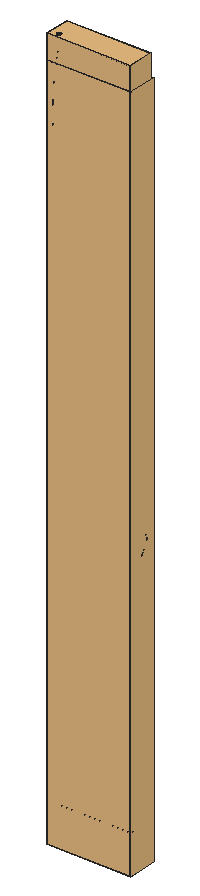
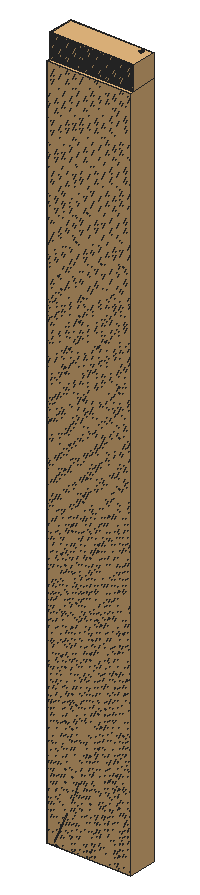
# SketchUp Ruby script. Lengths in inches.
U = 1.inch
M = Sketchup.active_model
def pt(a) = Geom::Point3d.new(a.map { |v| v * U })
def face(e, loops, mat)
  f = e.add_face(loops[0].map { |a| pt(a) })
  loops[1..].each { |l| e.add_face(l.map { |a| pt(a) }).erase! }
  f.material = f.back_material = mat if mat
  f
end
# faces: each face lists its corners as indices into pts; further lists are holes
def faces(e, pts, list, mat = nil) = list.each { |f| face(e, (f[0].is_a?(Array) ? f : [f]).map { |l| l.map { |i| pts[i] } }, mat) }
# xy, xz, yz: faces in a plane at the given z, y or x. An outline is a flat list of corners, or four numbers for a rectangle; further outlines are holes
def ring(l) = l.size == 4 ? [[l[0], l[1]], [l[2], l[1]], [l[2], l[3]], [l[0], l[3]]] : l.each_slice(2).to_a
def flat(e, list, mat, &to3) = list.each { |f| face(e, (f[0].is_a?(Array) ? f : [f]).map { |l| ring(l).map { |u, v| to3.(u, v) } }, mat) }
def xy(e, z, list, mat = nil) = flat(e, list, mat) { |x, y| [x, y, z] }
def xz(e, y, list, mat = nil) = flat(e, list, mat) { |x, z| [x, y, z] }
def yz(e, x, list, mat = nil) = flat(e, list, mat) { |y, z| [x, y, z] }
def lines(e, pts, list) = list.each { |a, b| e.add_line(pt(pts[a]), pt(pts[b])) }
# prism: a flat outline (further loops are holes) pulled along v
def prism(e, loops, v, mat = nil)
  f = face(e, loops, mat); d = Geom::Vector3d.new(v.map { |x| x * U })
  f.pushpull(f.normal.samedirection?(d) ? d.length : -d.length)
end
def box(e, o, s, mat = nil) = prism(e, [[o, [o[0] + s[0], o[1], o[2]], [o[0] + s[0], o[1] + s[1], o[2]], [o[0], o[1] + s[1], o[2]]]], [0, 0, s[2]], mat)
def at(x, y, z, deg = 0) = Geom::Transformation.translation(pt([x, y, z])) * Geom::Transformation.rotation(ORIGIN, Z_AXIS, deg.degrees)
def axes(o, x, y, z) = Geom::Transformation.new([*x, 0, *y, 0, *z, 0, *pt(o).to_a, 1])
def part(name) = M.definitions.add(name)
# library, detail: a bought-in or finely detailed component or shape, given as its bounding box
def library(name, o, s) = part(name).tap { |d| box(d.entities, o, s) }
def detail(e, o, s) = box(e.add_group.entities, o, s)
def put(e, d, t, mat = nil) = e.add_instance(d, t).tap { |i| i.material = mat if mat }
def group(e, t, mat = nil) = e.add_group.tap { |g| g.transformation = t; g.material = mat if mat }.entities
root = M.entities
M.materials.add("green").color = [174, 139, 102]
c1 = library("3DGeom~169_Defintion",[-36.08,-38.12,-500],[72.16,76.24,1000])
c2 = part("3DGeom~170_Defintion")
p = [[22.63,21.29,-499.8],[10.94,15.58,-499.92],[15.89,19.76,-500],[22.63,21.29,-499.8],[9.12,9.86,-499.6],[10.94,15.58,-499.92],
  [22.63,21.29,-499.8],[22.56,-1.57,-498.16],[15.83,-0.04,-498.58],[22.63,21.29,-499.8],[29.3,-0.04,-497.96],[22.56,-1.57,-498.16],
  [22.63,21.29,-499.8],[15.83,-0.04,-498.58],[10.91,4.15,-499.1],[22.63,21.29,-499.8],[34.25,4.15,-498.04],[29.3,-0.04,-497.96],
  [22.63,21.29,-499.8],[10.91,4.15,-499.1],[9.12,9.86,-499.6],[22.63,21.29,-499.8],[36.08,9.86,-498.37],[34.25,4.15,-498.04],
  [22.63,21.29,-499.8],[34.29,15.58,-498.86],[36.08,9.86,-498.37],[22.63,21.29,-499.8],[29.37,19.76,-499.39],[34.29,15.58,-498.86],
  [-22.3,-38.12,487.14],[-22.89,-17.99,500],[-34.125,-33.09,489.82],[-22.3,-38.12,487.14],[-34.125,-33.09,489.82],[-29.08,-36.77,487.69],
  [-10.78,-33.09,490.89],[-22.89,-17.99,500],[-22.3,-38.12,487.14],[-10.78,-33.09,490.89],[-22.3,-38.12,487.14],[-15.6,-36.77,488.31],
  [-34.125,-33.09,489.82],[-34.42,-23.02,496.25],[-36.08,-28.06,492.96],[-34.125,-33.09,489.82],[-22.89,-17.99,500],[-34.42,-23.02,496.25],
  [-11.07,-23.02,497.32],[-22.89,-17.99,500],[-10.78,-33.09,490.89],[-11.07,-23.02,497.32],[-10.78,-33.09,490.89],[-9.12,-28.06,494.18],
  [-22.89,-17.99,500],[-29.59,-19.34,498.83],[-34.42,-23.02,496.25],[-22.89,-17.99,500],[-11.07,-23.02,497.32],[-16.11,-19.34,499.45]]
faces(c2.entities,p,[[0,1,2],[3,4,5],[6,7,8],[9,10,11],[12,13,14],[15,16,17],[18,19,20],[21,22,23],
  [24,25,26],[27,28,29],[30,31,32],[33,34,35],[36,37,38],[39,40,41],[42,43,44],[45,46,47],
  [48,49,50],[51,52,53],[54,55,56],[57,58,59]],"green")
c3 = library("3DGeom~69_Defintion",[-21.55,-528.54,-60.47],[37.16,1000,121.53])
c4 = library("3DGeom~67_Defintion",[-21.08,-482.92,-59.16],[42.16,1000,118.9])
c5 = library("3DGeom~72_Defintion",[-21.55,-528.54,-60.94],[37.16,1000,122])
c6 = library("3DGeom~71_Defintion",[-21.08,-482.92,-59.62],[42.16,1000,119.36])
c7 = part("3DGeom~73_Defintion")
p = [[11.99,496.51,-49.8],[15.53,496.29,-49.63],[13.73,496.34,-49.94],[11.99,496.51,-49.8],[19.55,496.875,-46.43],[15.53,496.29,-49.63],
  [8.98,497.16,-48.31],[19.55,496.875,-46.43],[11.99,496.51,-49.8],[8.98,497.16,-48.31],[11.99,496.51,-49.8],[10.38,496.79,-49.24],
  [15.53,496.29,-49.63],[19.55,496.875,-46.43],[18.54,496.57,-47.79],[15.53,496.29,-49.63],[18.54,496.57,-47.79],[17.18,496.37,-48.89],
  [7.13,498.09,-45.48],[19.55,496.875,-46.43],[8.98,497.16,-48.31],[7.13,498.09,-45.48],[8.98,497.16,-48.31],[7.87,497.6,-47.04],
  [7.06,499.03,-42.12],[19.55,496.875,-46.43],[7.13,498.09,-45.48],[8.7,499.72,-39.2],[19.55,496.875,-46.43],[7.06,499.03,-42.12],
  [11.72,500,-37.36],[19.55,496.875,-46.43],[8.7,499.72,-39.2],[15.25,499.78,-37.19],[19.55,496.875,-46.43],[11.72,500,-37.36],
  [20.18,497.26,-44.875],[19.55,496.875,-46.43],[15.25,499.78,-37.19],[7.06,499.03,-42.12],[7.13,498.09,-45.48],[6.86,498.58,-43.78],
  [20.18,497.26,-44.875],[15.25,499.78,-37.19],[16.86,499.5,-37.75],[19.37,498.7,-39.95],[20.18,497.26,-44.875],[16.86,499.5,-37.75],
  [20.11,498.2,-41.51],[20.18,497.26,-44.875],[19.37,498.7,-39.95],[20.11,498.2,-41.51],[20.38,497.71,-43.21],[20.18,497.26,-44.875],
  [8.7,499.72,-39.2],[7.06,499.03,-42.12],[7.6875,499.41,-40.5625],[19.37,498.7,-39.95],[16.86,499.5,-37.75],[18.26,499.13,-38.68],
  [11.72,500,-37.36],[8.7,499.72,-39.2],[10.0625,499.92,-38.11],[15.25,499.78,-37.19],[11.72,500,-37.36],[13.51,499.95,-37.05],
  [-14.64,-499.34,43.17],[-13.98,-499.3,43.1],[-13.3,-499.28,43.21],[-15.79,-499.47,43.77],[-15.26,-499.4,43.4],[-14.64,-499.34,43.17],
  [-15.79,-499.47,43.77],[-14.64,-499.34,43.17],[-11.78,-499.375,44.44],[-14.64,-499.34,43.17],[-13.3,-499.28,43.21],[-11.78,-499.375,44.44],
  [-13.3,-499.28,43.21],[-12.16,-499.32,43.91],[-11.78,-499.375,44.44],[-13.3,-499.28,43.21],[-12.68,-499.29,43.49],[-12.16,-499.32,43.91],
  [-16.49,-499.66,44.89],[-16.21,-499.56,44.28],[-15.79,-499.47,43.77],[-16.49,-499.66,44.89],[-15.79,-499.47,43.77],[-11.78,-499.375,44.44],
  [-15.9,-499.96,47.36],[-16.52,-499.84,46.22],[-11.78,-499.375,44.44],[-14.76,-500,48.06],[-15.9,-499.96,47.36],[-11.78,-499.375,44.44],
  [-13.42,-499.94,48.1],[-14.76,-500,48.06],[-11.78,-499.375,44.44],[-11.54,-499.44,45.05],[-13.42,-499.94,48.1],[-11.78,-499.375,44.44],
  [-16.52,-499.84,46.22],[-16.49,-499.66,44.89],[-11.78,-499.375,44.44],[-16.52,-499.84,46.22],[-16.6,-499.75,45.57],[-16.49,-499.66,44.89],
  [-11.54,-499.44,45.05],[-12.81,-499.88,47.87],[-13.42,-499.94,48.1],[-11.85,-499.72,46.99],[-12.81,-499.88,47.87],[-11.54,-499.44,45.05],
  [-11.54,-499.44,45.05],[-11.57,-499.625,46.375],[-11.85,-499.72,46.99],[-11.54,-499.44,45.05],[-11.47,-499.53,45.7],[-11.57,-499.625,46.375],
  [-15.9,-499.96,47.36],[-16.28,-499.91,46.83],[-16.52,-499.84,46.22],[-11.85,-499.72,46.99],[-12.28,-499.81,47.5],[-12.81,-499.88,47.87],
  [-14.76,-500,48.06],[-15.39,-499.99,47.78],[-15.9,-499.96,47.36],[-13.42,-499.94,48.1],[-14.08,-499.98,48.17],[-14.76,-500,48.06]]
faces(c7.entities,p,[[0,1,2],[3,4,5],[6,7,8],[9,10,11],[12,13,14],[15,16,17],[18,19,20],[21,22,23],
  [24,25,26],[27,28,29],[30,31,32],[33,34,35],[36,37,38],[39,40,41],[42,43,44],[45,46,47],
  [48,49,50],[51,52,53],[54,55,56],[57,58,59],[60,61,62],[63,64,65],[66,67,68],[69,70,71],
  [72,73,74],[75,76,77],[78,79,80],[81,82,83],[84,85,86],[87,88,89],[90,91,92],[93,94,95],
  [96,97,98],[99,100,101],[102,103,104],[105,106,107],[108,109,110],[111,112,113],[114,115,116],[117,118,119],
  [120,121,122],[123,124,125],[126,127,128],[129,130,131]],"green")
c8 = part("3DGeom~70_Defintion")
p = [[4.6,125.58,-54.99],[6.02,125.73,-55.08],[7.6875,102.54,-61.3],[6.29,102.51,-61.18],[7.47,125.74,-54.81],[10.41,102.59,-60.39],
  [9.11,102.57,-61.03],[8.81,125.62,-54.19],[6.35,78.48,-56.16],[7.72,78.43,-56.26],[6.76,55.42,-43.45],[5.41,55.51,-43.38],
  [9.12,78.48,-56],[9.39,55.7,-42.65],[8.13,55.48,-43.2],[10.4,78.64,-55.4],[-1.7,166.83,-22.75],[3.1,146.54,-40.72],
  [1.67,146.34,-40.66],[-0.23,167.03,-22.81],[1.28,167.03,-22.54],[5.96,146.36,-39.87],[4.58,146.55,-40.45],[2.68,166.82,-21.96],
  [5.96,146.36,-39.87],[9.33,-111.73,-33.88],[9.98,-135.53,-35.71],[8.86,-135.47,-35.6],[10.48,-111.6875,-33.99],[11.65,-111.71,-33.79],
  [12.19,-135.57,-35.03],[11.13,-135.5625,-35.52],[12.73,-111.79,-33.3],[7.02,470.09,-31.89],[8.82,469.93,-32.05],[4.01,417.0625,-15.03],
  [2.26,417.2,-14.87],[10.67,469.875,-31.73],[7.47,417.07,-13.96],[5.8125,417.02,-14.72],[12.38,469.95,-30.95],[6.2,-163.01,-28.36],
  [7.28,-163.14,-28.46],[2.87,-193.54,-14.96],[1.83,-193.4,-14.88],[8.4,-163.1875,-28.26],[4.95,-193.56,-14.33],[3.95,-193.6,-14.77],
  [9.43,-163.16,-27.8],[3.97,33.4,-26.78],[3.77,12.01,-10.1],[2.48,12.11,-10.04],[5.29,33.3,-26.84],[6.64,33.37,-26.6],
  [6.31,12.3,-9.34],[5.1,12.08,-9.87],[7.88,33.6,-26.08],[6.31,12.3,-9.34],[6.08,-75.06,-12.84],[9.32,-91.88,-25.1],
  [8.16,-92,-25.02],[7.26,-74.91,-12.89],[8.47,-74.91,-12.67],[11.62,-92.03,-24.42],[10.52,-91.89,-24.9],[9.59,-75.0625,-12.2],
  [-6.88,214.4375,8.1875],[-3.27,189.12,-5.31],[-4.77,188.95,-5.22],[-5.35,214.53,8.05],[-3.78,214.51,8.32],[-0.3125,188.92,-4.43],
  [-1.73,189.11,-5.04],[-2.34,214.39,8.98],[-1.56,368.26,-1.78],[0.14,368.15,-1.9375],[-2.78,323.18,7.23],[-4.44,323.27,7.38],
  [1.89,368.1,-1.64],[0.48,323.17,8.24],[-1.09,323.15,7.51],[3.51,368.15,-0.9],[1.9375,-43.9375,7.47],[4.99,-59.32,-0.96],
  [3.79,-59.47,-0.91],[3.16,-43.83,7.38],[4.41,-43.82,7.62],[7.36,-59.44,-0.24],[6.22,-59.31,-0.74],[5.56,-43.88,8.17],
  [-3.44,-225.87,1.98],[-2.43,-226.02,1.91],[-7.8,-259.66,19.34],[-8.78,-259.53,19.41],[-1.39,-226.07,2.09],[-5.86,-259.67,19.92],
  [-6.8,-259.71,19.51],[-0.42,-226.02,2.52],[1.375,-8.2,3.21],[2.65,-8.27,3.13],[2.32,-27.1,9.4375],[1.07,-27.1,9.54],
  [3.94,-8.21,3.375],[4.75,-27.02,10.26],[3.59,-27.07,9.68],[5.13,-8.04,3.92],[-6.38,282.24,12.63],[-4.77,282.19,12.47],
  [-5.82,245.1875,13.79],[-7.38,245.2,13.95],[-3.125,282.16,12.75],[-2.76,245.14,14.75],[-4.22,245.17,14.07],[-1.61,282.16,13.46],
  [-13.375,-293.42,34.59],[-12.43,-293.53,34.5],[-15.51,-326.61,44.62],[-16.42,-326.55,44.71],[-11.46,-293.57,34.67],[-13.71,-326.61,45.16],
  [-14.57,-326.63,44.77],[-10.5625,-293.53,35.07],[-17.5,-495.0625,51.1],[-16.76,-495.03,51.03],[-14.84,-529.87,45.74],[-15.54,-529.91,45.81],
  [-16,-495.02,51.15],[-13.45,-529.86,46.16],[-14.12,-529.85,45.85],[-15.3,-495.03,51.46],[-18.08,-359.49,50.37],[-17.2,-359.53,50.28],
  [-18.18,-392.83,53.75],[-19.02,-392.8125,53.84],[-16.3,-359.54,50.42],[-16.51,-392.83,54.25],[-17.31,-392.83,53.89],[-15.47,-359.53,50.8],
  [-19.23,-426.52,55.12],[-18.43,-426.51,55.03],[-17.95,-460.58,54.125],[-18.73,-460.6,54.21],[-17.6,-426.51,55.16],[-16.43,-460.58,54.58],
  [-17.16,-460.57,54.25],[-16.83,-426.51,55.51]]
faces(c8.entities,p,[[0,1,2],[0,2,3],[4,5,6],[4,7,5],[8,9,10],[8,10,11],[12,13,14],[12,15,13],
  [16,17,18],[16,19,17],[20,21,22],[20,23,24],[25,26,27],[25,28,26],[29,30,31],[29,32,30],
  [33,34,35],[33,35,36],[37,38,39],[37,40,38],[41,42,43],[41,43,44],[45,46,47],[45,48,46],
  [49,50,51],[49,52,50],[53,54,55],[53,56,57],[58,59,60],[58,61,59],[62,63,64],[62,65,63],
  [66,67,68],[66,69,67],[70,71,72],[70,73,71],[74,75,76],[74,76,77],[78,79,80],[78,81,79],
  [82,83,84],[82,85,83],[86,87,88],[86,89,87],[90,91,92],[90,92,93],[94,95,96],[94,97,95],
  [98,99,100],[98,100,101],[102,103,104],[102,105,103],[106,107,108],[106,108,109],[110,111,112],[110,113,111],
  [114,115,116],[114,116,117],[118,119,120],[118,121,119],[122,123,124],[122,124,125],[126,127,128],[126,129,127],
  [130,131,132],[130,132,133],[134,135,136],[134,137,135],[138,139,140],[138,140,141],[142,143,144],[142,145,143]],"green")
c9 = part("3DGeom~68_Defintion")
p = [[6.16,100.31,-59.87],[7.52,100.34,-59.98],[7.56,76.74,-55.05],[6.21,76.79,-54.96],[8.91,100.36,-59.72],[10.17,76.95,-54.21],
  [8.92,76.8,-54.8],[10.1875,100.38,-59.09],[1.63,143.2,-39.79],[5.89,123.02,-53.9],[4.5,122.88,-53.81],[3.04,143.39,-39.84],
  [4.48,143.4,-39.58],[8.62,122.92,-53.03],[7.31,123.04,-53.63],[5.83,143.21,-39.01],[12.45,515.58,-51.71],[14.26,515.4,-51.86],
  [8.63,459.82,-31.36],[6.87,459.98,-31.21],[16.12,515.35,-51.54],[12.12,459.84,-30.29],[10.44,459.77,-31.05],[17.84,515.4375,-50.76],
  [5.3,54.32,-42.45],[6.61,54.23,-42.52],[5.18,32.58,-26.27],[3.89,32.68,-26.21],[7.96,54.29,-42.28],[7.71,32.88,-25.52],
  [6.5,32.65,-26.03],[9.1875,54.5,-41.73],[7.71,32.88,-25.52],[8.67,-132.56,-34.83],[9.76,-132.61,-34.94],[7.13,-159.63,-27.84],
  [10.89,-132.65,-34.76],[9.23,-159.65,-27.2],[8.22,-159.68,-27.66],[6.07,-159.51,-27.75],[11.93,-132.65,-34.28],[7.99,-90.02,-24.49],
  [9.125,-89.91,-24.56],[10.25,-109.28,-33.26],[9.13,-109.32,-33.15],[10.29,-89.92,-24.36],[12.45,-109.39,-32.58],[11.4,-109.31,-33.07],
  [11.37,-90.05,-23.89],[-4.67,184.89,-5.11],[-0.23,163.4375,-22.32],[-1.66,163.24,-22.26],[-3.2,185.05,-5.19],[-1.7,185.04,-4.93],
  [2.62,163.24,-21.49],[1.25,163.44,-22.05],[-0.3,184.86,-4.34],[2.62,163.24,-21.49],[2.21,408.23,-14.55],[3.93,408.09,-14.7],
  [0.14,360.23,-1.9],[1.79,-189.24,-14.5625],[-2.375,-221.15,1.87],[-3.36,-221.01,1.9375],[2.8125,-189.38,-14.64],[-1.53,360.34,-1.74],
  [3.87,-189.4375,-14.46],[-0.41,-221.16,2.46],[-1.36,-221.21,2.05],[4.84,-189.4,-14.02],[5.6875,408.05,-14.4],[3.43,360.23,-0.88],
  [1.85,360.1875,-1.6],[7.3125,408.11,-13.66],[3.71,-58.1875,-0.89],[7.1,-73.3,-12.61],[5.95,-73.45,-12.5625],[4.88,-58.04,-0.94],
  [6.08,-58.03,-0.72],[9.39,-73.45,-11.9375],[8.29,-73.3,-12.4],[7.2,-58.16,-0.23],[9.39,-73.45,-11.9375],[2.43,11.85,-9.83],
  [3.69,11.75,-9.89],[2.59,-8.09,3.07],[1.34,-8.02,3.15],[4.99,11.82,-9.66],[5.02,-7.87,3.83],[3.86,-8.04,3.3],
  [6.17,12.03,-9.14],[5.02,-7.87,3.83],[-4.34,316.32,7.22],[-2.72,316.23,7.07],[-4.67,276.12,12.2],[1.05,-26.51,9.34],
  [3.09,-42.89,7.22],[1.89,-42.99,7.31],[2.27,-26.51,9.24],[-6.24,276.17,12.36],[-1.0625,316.2,7.35],[-1.57,276.09,13.17],
  [-3.06,276.09,12.48],[0.47,316.22,8.0625],[3.52,-26.49,9.47],[5.44,-42.94,7.99],[4.32,-42.875,7.45],[-7.22,239.93,13.65],
  [-5.23,209.91,7.88],[-6.73,209.82,8.01],[-5.69,239.92,13.5],[4.65,-26.43,10.03],[-4.13,239.89,13.76],[-2.29,209.78,8.79],
  [-3.7,209.9,8.14],[-2.7,239.86,14.43],[-8.59,-253.95,18.99],[-7.64,-254.08,18.92],[-12.17,-287.22,33.76],[-13.09,-287.11,33.84],
  [-6.65,-254.125,19.09],[-10.33,-287.22,34.3125],[-11.21,-287.25,33.92],[-5.74,-254.08,19.49],[-16.07,-319.53,43.75],[-15.17,-319.59,43.66],
  [-16.83,-351.79,49.2],[-17.69,-351.76,49.29],[-14.26,-319.61,43.81],[-15.14,-351.79,49.71],[-15.95,-351.81,49.34],[-13.41,-319.59,44.19],
  [-18.32,-450.69,53.04],[-17.57,-450.68,52.96],[-16.4,-484.39,49.93],[-17.12,-484.42,50.01],[-16.79,-450.67,53.08],[-14.97,-484.38,50.36],
  [-15.66,-484.375,50.05],[-16.08,-450.67,53.41],[-18.61,-384.37,52.68],[-17.78,-384.38,52.59],[-18.03,-417.34,53.85],[-18.82,-417.34,53.93],
  [-16.9375,-384.39,52.73],[-16.47,-417.34,54.32],[-17.22,-417.34,53.98],[-16.16,-384.38,53.08]]
faces(c9.entities,p,[[0,1,2],[0,2,3],[4,5,6],[4,7,5],[8,9,10],[8,11,9],[12,13,14],[12,15,13],
  [16,17,18],[16,18,19],[20,21,22],[20,23,21],[24,25,26],[24,26,27],[28,29,30],[28,31,32],
  [33,34,35],[36,37,38],[33,35,39],[36,40,37],[41,42,43],[41,43,44],[45,46,47],[45,48,46],
  [49,50,51],[49,52,50],[53,54,55],[53,56,57],[58,59,60],[61,62,63],[61,64,62],[58,60,65],
  [66,67,68],[66,69,67],[70,71,72],[70,73,71],[74,75,76],[74,77,75],[78,79,80],[78,81,82],
  [83,84,85],[83,85,86],[87,88,89],[87,90,91],[92,93,94],[95,96,97],[95,98,96],[92,94,99],
  [100,101,102],[100,103,101],[104,105,106],[107,108,109],[107,110,108],[104,111,105],[112,113,114],[112,115,113],
  [116,117,118],[116,118,119],[120,121,122],[120,123,121],[124,125,126],[124,126,127],[128,129,130],[128,131,129],
  [132,133,134],[132,134,135],[136,137,138],[136,139,137],[140,141,142],[140,142,143],[144,145,146],[144,147,145]],"green")
c10 = part("3DGeom~66_Defintion")
p = [[6.02,125.75,-55.09],[9.11,102.59,-61.04],[7.6875,102.5625,-61.3125],[7.47,125.77,-54.82],[7.72,78.45,-56.27],[8.13,55.5,-43.21],
  [6.76,55.43,-43.46],[9.12,78.5,-56.01],[-0.23,167.06,-22.8125],[4.58,146.58,-40.46],[3.1,146.57,-40.73],[1.28,167.07,-22.54],
  [10.48,-111.71,-34],[11.13,-135.59,-35.53],[9.98,-135.56,-35.72],[11.65,-111.73,-33.8],[8.82,470.02,-32.05],[5.8125,417.1,-14.72],
  [4.01,417.15,-15.03],[10.68,469.97,-31.74],[7.29,-163.17,-28.46],[3.95,-193.64,-14.78],[2.875,-193.58,-14.96],[8.4,-163.22,-28.27],
  [5.29,33.31,-26.85],[5.1,12.08,-9.87],[3.78,12.01,-10.11],[6.64,33.37,-26.61],[7.26,-74.92,-12.89],[10.52,-91.91,-24.9],
  [9.33,-91.9,-25.11],[8.47,-74.92,-12.68],[-5.35,214.57,8.06],[-1.73,189.15,-5.04],[-3.27,189.15,-5.31],[-3.78,214.56,8.32],
  [0.14,368.22,-1.9375],[-1.09,323.22,7.52],[-2.78,323.25,7.23],[1.89,368.18,-1.64],[3.16,-43.84,7.38],[6.22,-59.32,-0.74],
  [4.99,-59.33,-0.96],[4.41,-43.82,7.62],[-2.43,-226.0625,1.91],[-6.8,-259.76,19.51],[-7.8,-259.72,19.34],[-1.39,-226.12,2.09],
  [2.65,-8.27,3.13],[3.59,-27.07,9.68],[2.32,-27.1,9.44],[3.94,-8.22,3.375],[-4.77,282.25,12.47],[-4.22,245.22,14.07],
  [-5.82,245.24,13.8],[-3.125,282.22,12.75],[-12.4375,-293.59,34.51],[-14.57,-326.7,44.78],[-15.51,-326.68,44.63],[-11.46,-293.625,34.67],
  [-16.76,-495.13,51.04],[-14.12,-529.96,45.86],[-14.84,-529.98,45.75],[-16,-495.12,51.16],[-17.21,-359.6,50.29],[-17.3125,-392.91,53.9],
  [-18.18,-392.91,53.76],[-16.3,-359.61,50.43],[-18.43,-426.6,55.04],[-17.16,-460.67,54.26],[-17.96,-460.68,54.13],[-17.6,-426.6,55.17]]
faces(c10.entities,p,[[0,1,2],[0,3,1],[4,5,6],[4,7,5],[8,9,10],[8,11,9],[12,13,14],[12,15,13],
  [16,17,18],[16,19,17],[20,21,22],[20,23,21],[24,25,26],[24,27,25],[28,29,30],[28,31,29],
  [32,33,34],[32,35,33],[36,37,38],[36,39,37],[40,41,42],[40,43,41],[44,45,46],[44,47,45],
  [48,49,50],[48,51,49],[52,53,54],[52,55,53],[56,57,58],[56,59,57],[60,61,62],[60,63,61],
  [64,65,66],[64,67,65],[68,69,70],[68,71,69]],"green")
c11 = part("3DGeom~65_Defintion")
p = [[7.52,100.36,-59.99],[8.92,100.38,-59.73],[8.93,76.8125,-54.81],[7.56,76.76,-55.0625],[3.04,143.42,-39.85],[7.31,123.06,-53.64],
  [5.89,123.05,-53.91],[4.49,143.43,-39.59],[14.26,515.51,-51.87],[10.45,459.87,-31.05],[8.63,459.92,-31.36],[16.125,515.46,-51.55],
  [6.62,54.24,-42.53],[6.5,32.65,-26.04],[5.18,32.59,-26.27],[7.96,54.3,-42.28],[9.77,-132.64,-34.95],[8.22,-159.71,-27.66],
  [7.13,-159.66,-27.85],[10.89,-132.67,-34.76],[9.125,-89.93,-24.57],[11.4,-109.33,-33.07],[10.25,-109.31,-33.26],[10.29,-89.9375,-24.36],
  [-3.2,185.09,-5.2],[1.25,163.47,-22.06],[-0.23,163.47,-22.32],[-1.7,185.08,-4.93],[3.93,408.18,-14.71],[1.85,360.26,-1.6],
  [0.14,360.3,-1.9],[5.6875,408.13,-14.4],[2.8125,-189.42,-14.64],[-1.36,-221.25,2.05],[-2.375,-221.2,1.87],[3.87,-189.48,-14.46],
  [4.88,-58.05,-0.94],[8.29,-73.3125,-12.4],[7.1,-73.3125,-12.62],[6.08,-58.04,-0.72],[3.69,11.76,-9.89],[3.86,-8.04,3.3],
  [2.59,-8.09,3.07],[4.99,11.82,-9.66],[-2.72,316.3,7.07],[-3.06,276.15,12.48],[-4.67,276.18,12.21],[-1.0625,316.27,7.35],
  [2.27,-26.52,9.24],[4.32,-42.88,7.46],[3.09,-42.9,7.22],[3.52,-26.49,9.47],[-5.7,239.97,13.5],[-3.7,209.94,8.14],
  [-5.24,209.96,7.88],[-4.13,239.94,13.77],[-7.64,-254.13,18.93],[-11.22,-287.3125,33.93],[-12.17,-287.28,33.77],[-6.65,-254.18,19.09],
  [-15.18,-319.65,43.67],[-15.95,-351.88,49.35],[-16.84,-351.87,49.21],[-14.26,-319.67,43.82],[-17.57,-450.77,52.97],[-15.66,-484.48,50.06],
  [-16.4,-484.49,49.94],[-16.79,-450.76,53.09],[-17.79,-384.46,52.6],[-17.22,-417.43,53.99],[-18.03,-417.43,53.86],[-16.94,-384.47,52.74]]
faces(c11.entities,p,[[0,1,2],[0,2,3],[4,5,6],[4,7,5],[8,9,10],[8,11,9],[12,13,14],[12,15,13],
  [16,17,18],[16,19,17],[20,21,22],[20,23,21],[24,25,26],[24,27,25],[28,29,30],[28,31,29],
  [32,33,34],[32,35,33],[36,37,38],[36,39,37],[40,41,42],[40,43,41],[44,45,46],[44,47,45],
  [48,49,50],[48,51,49],[52,53,54],[52,55,53],[56,57,58],[56,59,57],[60,61,62],[60,63,61],
  [64,65,66],[64,67,65],[68,69,70],[68,71,69]],"green")
c12 = library("3DGeom~90_Defintion",[-21.63,-500,-162.35],[43.26,1000,324.7])
c13 = part("3DGeom~91_Defintion")
p = [[4.77,500,-131.64],[5.88,490.68,-162.35],[-2.34,491.3,-160.59],[4.77,500,-131.64],[13.96,491.3,-160],[5.88,490.68,-162.35],
  [4.77,500,-131.64],[-2.34,491.3,-160.59],[-8.52,493.01,-155.1875],[4.77,500,-131.64],[19.73,493.01,-154.16],[13.96,491.3,-160],
  [4.77,500,-131.64],[-8.52,493.01,-155.1875],[-10.98,495.34,-147.59],[4.77,500,-131.64],[21.63,495.34,-146.41],[19.73,493.01,-154.16],
  [4.77,500,-131.64],[-10.98,495.34,-147.59],[-9.08,497.67,-139.83],[4.77,500,-131.64],[19.17,497.67,-138.81],[21.63,495.34,-146.41],
  [4.77,500,-131.64],[-9.08,497.67,-139.83],[-3.3125,499.375,-134],[4.77,500,-131.64],[13,499.375,-133.4],[19.17,497.67,-138.81],
  [-4.37,-494.09,119.72],[-5.53,-500,151.58],[-18.78,-495.57,127.17],[9.46,-495.57,128.2],[-5.53,-500,151.58],[-4.37,-494.09,119.72],
  [-4.37,-494.09,119.72],[-18.78,-495.57,127.17],[-12.6,-494.49,121.56],[9.46,-495.57,128.2],[-4.37,-494.09,119.72],[3.71,-494.49,122.15],
  [-18.78,-495.57,127.17],[-5.53,-500,151.58],[-19.36,-498.52,143.1],[-18.78,-495.57,127.17],[-19.36,-498.52,143.1],[-21.25,-497.04,135.06],
  [8.89,-498.52,144.13],[-5.53,-500,151.58],[9.46,-495.57,128.2],[8.89,-498.52,144.13],[9.46,-495.57,128.2],[11.36,-497.04,136.24],
  [-5.53,-500,151.58],[-13.6,-499.6,149.15],[-19.36,-498.52,143.1],[-5.53,-500,151.58],[8.89,-498.52,144.13],[2.7,-499.6,149.74]]
faces(c13.entities,p,[[0,1,2],[3,4,5],[6,7,8],[9,10,11],[12,13,14],[15,16,17],[18,19,20],[21,22,23],
  [24,25,26],[27,28,29],[30,31,32],[33,34,35],[36,37,38],[39,40,41],[42,43,44],[45,46,47],
  [48,49,50],[51,52,53],[54,55,56],[57,58,59]],"green")
g1 = group(root,at(15.3125,38.42,26.21))
put(g1,c1,axes([-1.27,0.04,6.98],[0,0.0011,0],[0,0,-0.0011],[-0.0011,0,0]),"green")
put(g1,c2,axes([-1.27,0.04,6.98],[0,0.0011,0],[0,0,-0.0011],[-0.0011,0,0]),"green")
put(root,c3,axes([14.0625,38.4,36.46],[0,0.01017,0],[0,0,-0.01017],[-0.01017,0,0]),"green")
put(root,c4,axes([14.0625,38.4,36.46],[0,0.0104,0],[0,0,-0.0104],[-0.0104,0,0]),"green")
put(root,c5,axes([14.0625,38.4,36.46],[0,0.01017,0],[0,0,-0.01017],[-0.01017,0,0]),"green")
put(root,c6,axes([14.0625,38.4,36.46],[0,0.0104,0],[0,0,-0.0104],[-0.0104,0,0]),"green")
put(root,c7,axes([14.0625,38.4,36.46],[0,0.01076,0],[0,0,-0.01076],[-0.01076,0,0]),"green")
put(root,c8,axes([14.0625,38.4,36.46],[0,0.01013,0],[0,0,-0.01013],[-0.01013,0,0]),"green")
put(root,c9,axes([14.0625,38.4,36.46],[0,0.01036,0],[0,0,-0.01036],[-0.01036,0,0]),"green")
put(root,c10,axes([14.0625,38.4,36.46],[0,0.01013,0],[0,0,-0.01013],[-0.01013,0,0]),"green")
put(root,c11,axes([14.0625,38.4,36.46],[0,0.01036,0],[0,0,-0.01036],[-0.01036,0,0]),"green")
g2 = group(root,at(15.3125,38.42,26.21))
put(g2,c12,axes([-1.19,0.04,6.22],[0,0.00091,0],[0,0,-0.00091],[-0.00091,0,0]),"green")
put(g2,c13,axes([-1.19,0.04,6.22],[0,0.00091,0],[0,0,-0.00091],[-0.00091,0,0]),"green")
